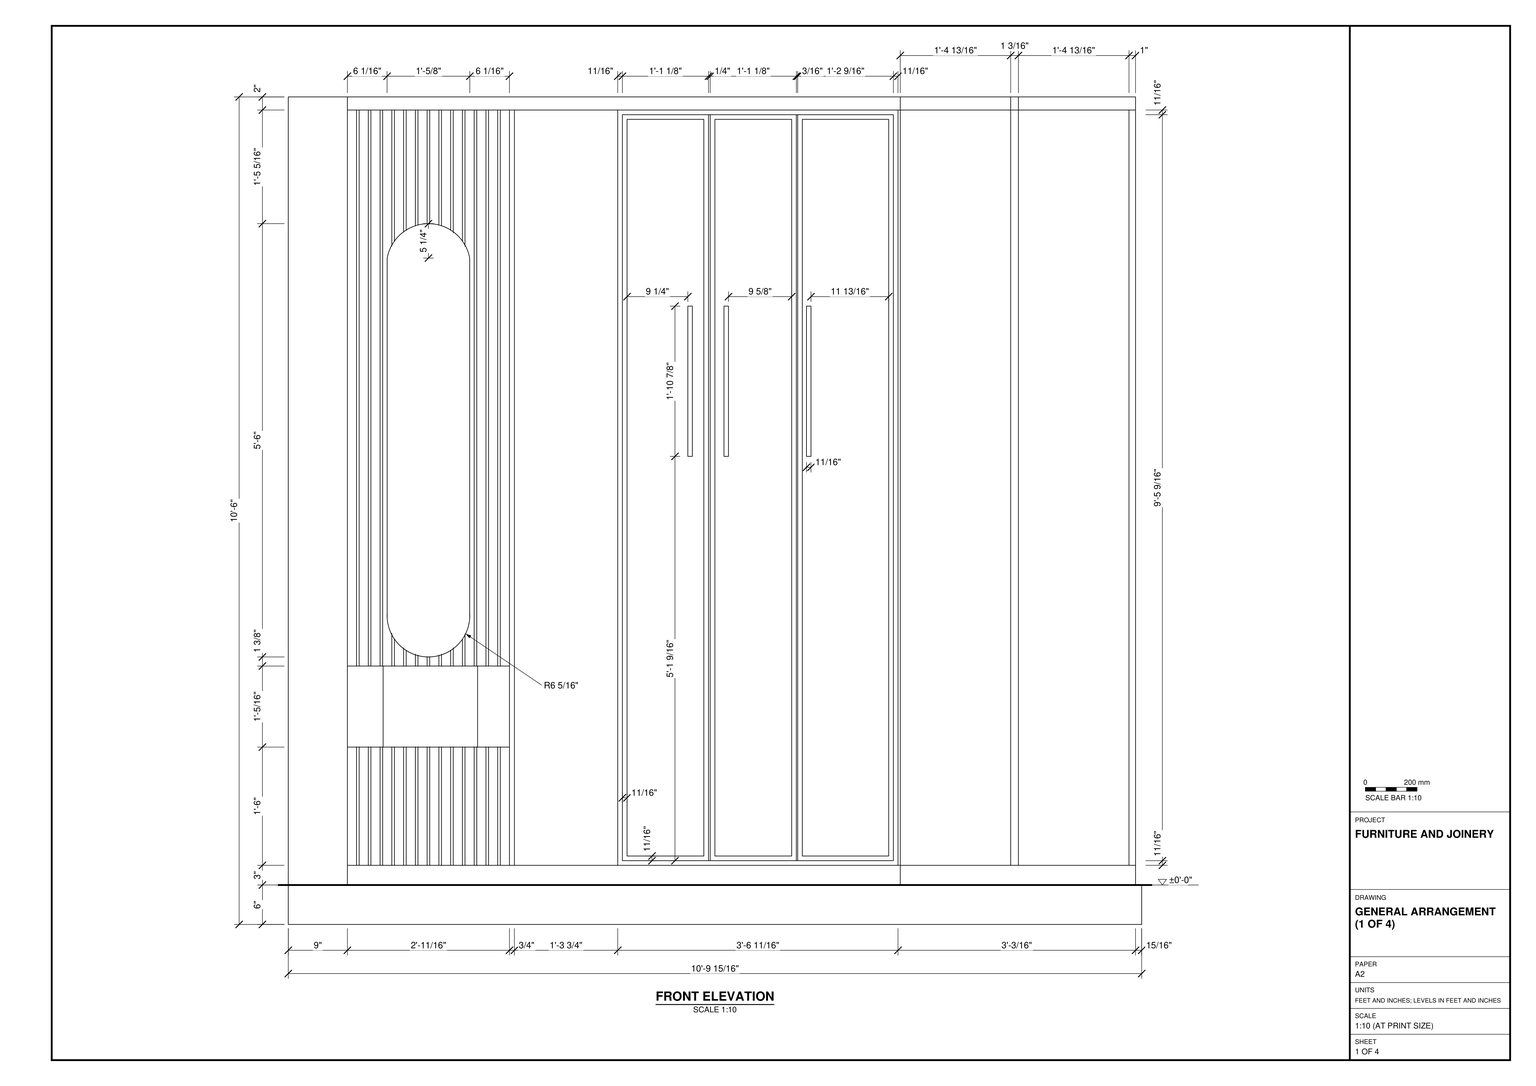
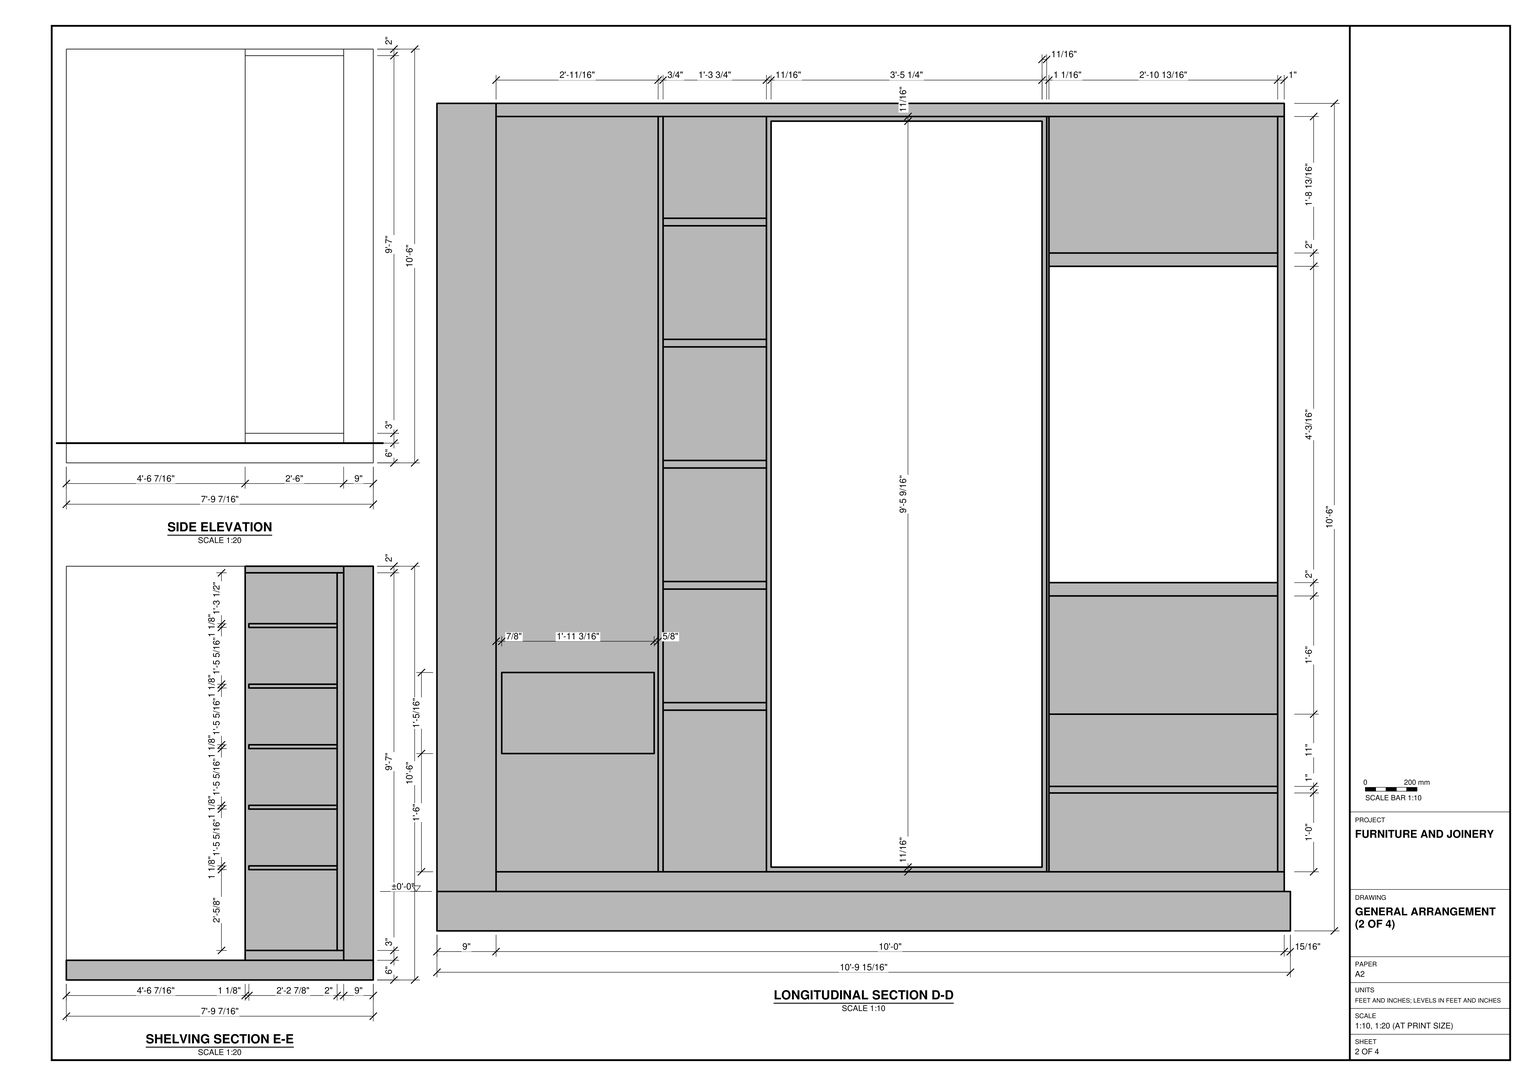
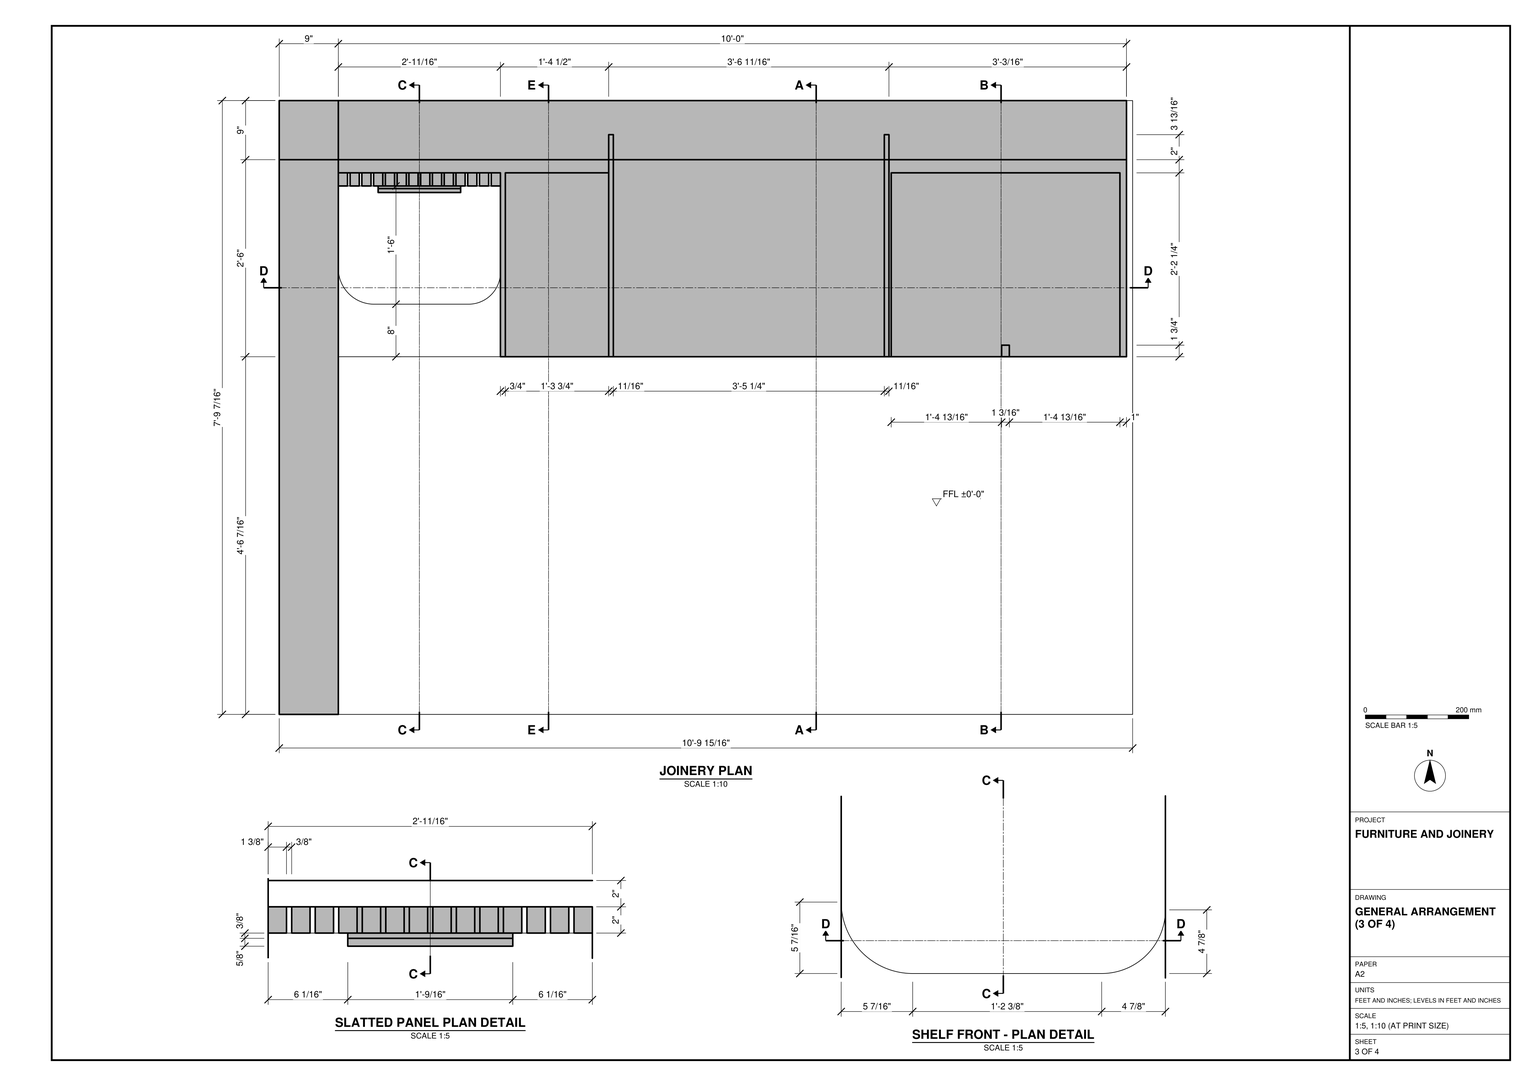
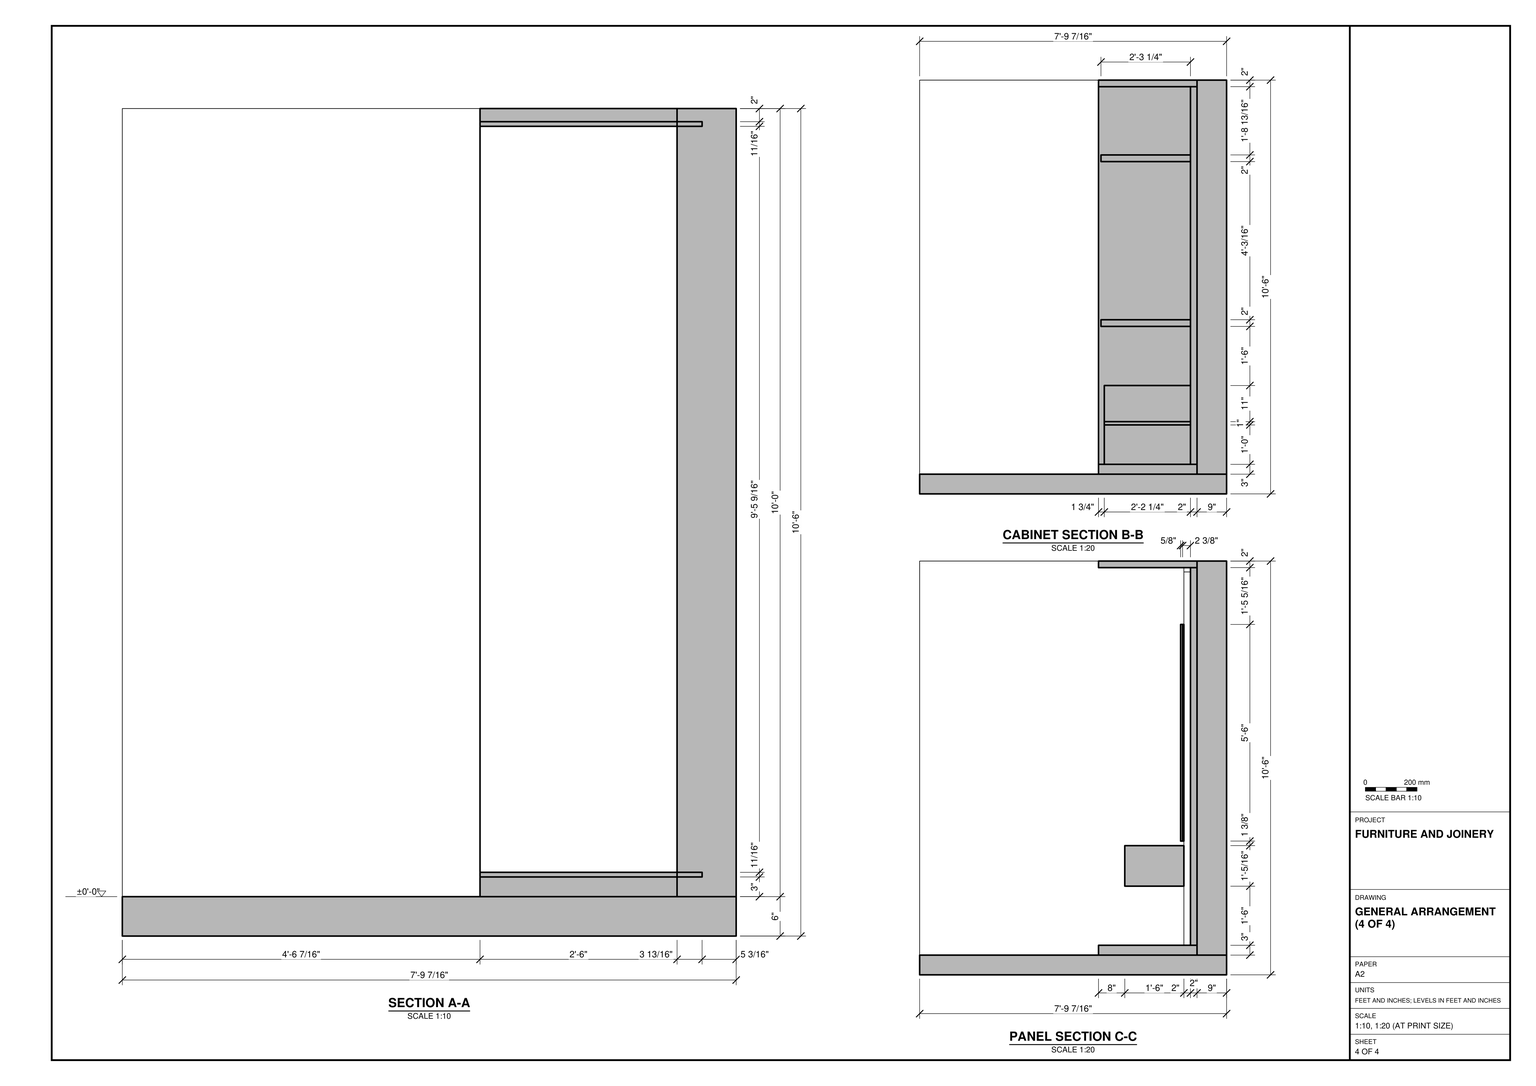
Build the wardrobe and its surrounding wall corner in SketchUp using task_files/diagram_01.pdf. Work in feet and inches, with the finished floor at ±0'-0". Including the floor slab and walls, the model measures 10'-9 15/16" wide, 7'-9 7/16" deep and 10'-6" high. Model the 6" floor slab and the 9" rear and left walls. Set the 10'-0" joinery run against the rear wall, starting at the inside face of the left wall, and leave the floor in front clear as shown in plan.

Build the continuous plinth and top panel. At the left end, centre the tall, round-ended mirror on the vertical slats. Fit the projecting shelf below it, following the plan detail for its rounded front corners. Between the mirror bay and the three framed wardrobe doors, build the narrow stack of shelves shown in section. Match the position of each door pull to the front elevation. In the right-hand bay, follow the elevation for the front divisions and the longitudinal section for the internal compartments.

Keep the slab, walls and distinct joinery pieces in separate groups or components, and use components for repeated parts. Any decor or loose items shown may be represented by suitable library components. Save one SketchUp model as output_files/wardrobe_with_shelving_and_mirrored_dressing_bay.skp.

# SketchUp Ruby script. Lengths in inches.
U = 1.inch
M = Sketchup.active_model
def pt(a) = Geom::Point3d.new(a.map { |v| v * U })
def face(e, loops, mat)
  f = e.add_face(loops[0].map { |a| pt(a) })
  loops[1..].each { |l| e.add_face(l.map { |a| pt(a) }).erase! }
  f.material = f.back_material = mat if mat
  f
end
# faces: each face lists its corners as indices into pts; further lists are holes
def faces(e, pts, list, mat = nil) = list.each { |f| face(e, (f[0].is_a?(Array) ? f : [f]).map { |l| l.map { |i| pts[i] } }, mat) }
# xy, xz, yz: faces in a plane at the given z, y or x. An outline is a flat list of corners, or four numbers for a rectangle; further outlines are holes
def ring(l) = l.size == 4 ? [[l[0], l[1]], [l[2], l[1]], [l[2], l[3]], [l[0], l[3]]] : l.each_slice(2).to_a
def flat(e, list, mat, &to3) = list.each { |f| face(e, (f[0].is_a?(Array) ? f : [f]).map { |l| ring(l).map { |u, v| to3.(u, v) } }, mat) }
def xy(e, z, list, mat = nil) = flat(e, list, mat) { |x, y| [x, y, z] }
def xz(e, y, list, mat = nil) = flat(e, list, mat) { |x, z| [x, y, z] }
def yz(e, x, list, mat = nil) = flat(e, list, mat) { |y, z| [x, y, z] }
def lines(e, pts, list) = list.each { |a, b| e.add_line(pt(pts[a]), pt(pts[b])) }
# prism: a flat outline (further loops are holes) pulled along v
def prism(e, loops, v, mat = nil)
  f = face(e, loops, mat); d = Geom::Vector3d.new(v.map { |x| x * U })
  f.pushpull(f.normal.samedirection?(d) ? d.length : -d.length)
end
def box(e, o, s, mat = nil) = prism(e, [[o, [o[0] + s[0], o[1], o[2]], [o[0] + s[0], o[1] + s[1], o[2]], [o[0], o[1] + s[1], o[2]]]], [0, 0, s[2]], mat)
def at(x, y, z, deg = 0) = Geom::Transformation.translation(pt([x, y, z])) * Geom::Transformation.rotation(ORIGIN, Z_AXIS, deg.degrees)
def axes(o, x, y, z) = Geom::Transformation.new([*x, 0, *y, 0, *z, 0, *pt(o).to_a, 1])
def part(name) = M.definitions.add(name)
# library, detail: a bought-in or finely detailed component or shape, given as its bounding box
def library(name, o, s) = part(name).tap { |d| box(d.entities, o, s) }
def detail(e, o, s) = box(e.add_group.entities, o, s)
def put(e, d, t, mat = nil) = e.add_instance(d, t).tap { |i| i.material = mat if mat }
def group(e, t, mat = nil) = e.add_group.tap { |g| g.transformation = t; g.material = mat if mat }.entities
root = M.entities
M.materials.add("[Color E01]").color = [255, 255, 204]
M.materials.add("[Color E03]").color = [255, 255, 101]
M.materials.add("[Color G01]").color = [204, 255, 204]
M.materials.add("[Metal Steel Textured]").color = [106, 110, 123]
M.materials.add("[Translucent Glass Gray]").color = [128, 128, 128]
M.materials["[Translucent Glass Gray]"].alpha = 0.5
c1 = part("Wardrobe shelf")
box(c1.entities,[0,-26.875,0],[15.73,26.875,1.15],"[Color E01]")
c2 = part("Wardrobe upright")
prism(c2.entities,[[[0,0,115],[1.4,0,115],[1.4,0,113.6875],[1.4,0,0],[0,0,0]]],[0,-2,0],"[Color E01]")
c3 = part("Group\#10")
xz(c3.entities,0,[[0,0,0.6875,22.875]])
c4 = library("Group\#11",[-0.02,-1,-1.38],[12.6,1,65.97])
g1 = group(root,at(3.61,0,0))
box(g1,[-3.61,0,0],[129.94,93.46,6])
g2 = group(root,at(9,84.46,6))
xy(g2,0,[[-9,-84.46,0,0],[-9,0,0,9],[0,0,120,9]])
xy(g2,120,[[-9,-84.46,0,0],[-9,0,0,9],[0,0,120,9]])
xz(g2,-84.46,[[-9,0,0,120]])
xz(g2,0,[[-9,0,0,120],[0,0,120,120]])
xz(g2,9,[[-9,0,0,120],[0,0,120,120]])
yz(g2,-9,[[-84.46,0,0,120],[0,0,9,120]])
yz(g2,0,[[-84.46,0,0,120],[0,0,9,120]])
yz(g2,120,[[0,0,9,120]])
g3 = group(root,at(9,60.46,6),"[Color E01]")
xy(g3,0,[[0,-6,120,24]],"[Color E03]")
xy(g3,3,[[100.99,-6,102.16,-4.24]])
xy(g3,3,[[0,-6,24.68,22],[25.43,-6,41.16,22],[41.16,24,83.84,27.8125]],"[Color E01]")
xy(g3,3,[[24.68,-6,25.43,-6,25.43,22,41.16,22,41.16,24,0,24,0,22,24.68,22],[41.16,-6,83.84,24],[83.84,-6,84.18,-6,84.18,22,119,22,119,-6,120,-6,120,24,83.84,24],[84.18,-6,100.99,-4.24],[102.16,-6,119,-4.24]],"[Color E03]")
xy(g3,3.71,[[41.87,-6,83.125,27.8125]],"[Color E01]")
xy(g3,117.29,[[41.87,-6,83.125,27.8125]],"[Color E01]")
xy(g3,118,[[0,-6,24.68,22],[25.43,-6,41.16,22],[84.18,-6,84.18,22,119,22,119,-6,102.16,-6,102.16,-4.24,100.99,-4.24,100.99,-6],[41.16,24,83.84,27.8125]],"[Color E01]")
xy(g3,118,[[24.68,-6,24.68,22,0,22,0,24,41.16,24,41.16,22,25.43,22,25.43,-6],[41.16,-6,83.84,24],[83.84,-6,83.84,24,120,24,120,-6,119,-6,119,22,84.18,22,84.18,-6]],"[Color E03]")
xy(g3,120,[[0,-6,120,24]],"[Color E01]")
xz(g3,-6,[[0,0,84.18,3],[84.18,0,120,3],[24.68,3,25.43,118],[[41.16,3,83.84,118],[54.98,3.71,83.125,117.29]],[83.84,3,84.18,118],
  [119,3,120,118],[54.98,3.71,83.125,117.29],[0,118,84.18,120],[84.18,118,100.99,120],[100.99,118,102.16,120],
  [102.16,118,120,120]],"[Color E01]")
xz(g3,-6,[[100.99,3,102.16,118]],"[Metal Steel Textured]")
xz(g3,-6,[[25.43,3,41.16,118],[84.18,3,100.99,118],[102.16,3,119,118]],"[Translucent Glass Gray]")
xz(g3,-4.24,[[100.99,3,102.16,118]],"[Color E03]")
xz(g3,22,[[0,3,23.28,118],[25.43,3,41.16,101.36],[84.18,3,119,45],[84.18,47.03,119,118],[25.43,102.51,41.16,118]],"[Color E01]")
xz(g3,24,[[0,0,120,3],[0,3,120,118],[0,118,120,120]],"[Color E03]")
xz(g3,27.8125,[[[41.16,3,83.84,118],[41.87,3.71,83.125,117.29]]],"[Color E01]")
yz(g3,0,[[-6,0,24,3],[22,3,24,118],[-6,118,24,120]],"[Color E01]")
yz(g3,24.68,[[-6,3,22,116.6875],[-6,116.6875,22,118]],"[Color E01]")
yz(g3,25.43,[[-6,3,22,118]],"[Color E01]")
yz(g3,41.16,[[-6,3,22,118],[22,3,27.8125,118]],"[Color E01]")
yz(g3,41.87,[[-6,3.71,27.8125,117.29]],"[Color E01]")
yz(g3,83.125,[[-6,3.71,27.8125,117.29]],"[Color E01]")
yz(g3,83.84,[[-6,3,27.8125,118]],"[Color E01]")
yz(g3,84.18,[[-6,3,22,118]],"[Color E01]")
yz(g3,100.99,[[-6,3,-4.24,118]],"[Color E03]")
yz(g3,102.16,[[-6,3,-4.24,118]],"[Color E03]")
yz(g3,119,[[-6,3,22,118]],"[Color E01]")
yz(g3,120,[[-6,3,24,118],[-6,118,24,120]],"[Color E01]")
yz(g3,120,[[-6,0,24,3]],"[Color E03]")
put(g3,c1,at(25.43,22,101.36))
put(g3,c1,at(25.43,22,82.92))
put(g3,c1,at(25.43,22,64.48))
put(g3,c1,at(25.43,22,46.04))
put(g3,c1,at(25.43,22,27.61))
put(g3,c2,at(23.28,22,3))
put(g3,c2,at(21.49,22,3))
put(g3,c2,at(19.7,22,3))
put(g3,c2,at(17.91,22,3))
put(g3,c2,at(16.12,22,3))
put(g3,c2,at(14.33,22,3))
put(g3,c2,at(12.54,22,3))
put(g3,c2,at(10.75,22,3))
put(g3,c2,at(8.95,22,3))
put(g3,c2,at(7.16,22,3))
put(g3,c2,at(5.37,22,3))
put(g3,c2,at(3.58,22,3))
put(g3,c2,at(1.79,22,3))
put(g3,c2,at(0,22,3))
g4 = group(g3,at(84.18,-4.24,3),"[Color E01]")
xy(g4,0,[[0,0,34.82,26.24]])
xy(g4,12,[[0,0,34.82,26.24]])
xy(g4,13,[[0,0,34.82,26.24]])
xy(g4,24,[[0,0,34.82,26.24]])
xz(g4,0,[[0,0,34.82,12],[0,12,34.82,13],[0,13,34.82,24]])
xz(g4,26.24,[[0,0,34.82,12],[0,12,34.82,13],[0,13,34.82,24]])
yz(g4,0,[[0,0,26.24,12],[0,12,26.24,13],[0,13,26.24,24]])
yz(g4,34.82,[[0,0,26.24,12],[0,12,26.24,13],[0,13,26.24,24]])
g5 = group(g3,at(84.18,22,45),"[Color E01]")
xy(g5,0,[[0,-27.25,34.82,0]],"[Color G01]")
xy(g5,2.03,[[0,-27.25,34.82,0]],"[Color E01]")
xz(g5,-27.25,[[0,0,34.82,2.03]],"[Color E01]")
xz(g5,0,[[0,0,34.82,2.03]],"[Color G01]")
yz(g5,0,[[-27.25,0,0,2.03]],"[Color G01]")
yz(g5,34.82,[[-27.25,0,0,2.03]],"[Color G01]")
g6 = group(g3,at(84.18,22,95.1875),"[Color E01]")
box(g6,[0,-27.25,0],[34.82,27.25,2.03],"[Color E01]")
put(g3,c3,at(51.83,-6,65.27))
put(g3,c3,at(57.33,-6,65.27))
put(g3,c3,at(69.9,-6,65.27))
g7 = group(g3,at(41.87,-6,3.71))
xz(g7,0,[[[0,0,13.11,113.58],[0.71,0.71,12.4,112.875]],[0.71,0.71,12.4,112.875]],"[Color E01]")
g8 = group(g3,at(55.25,-6,3.71))
xz(g8,0,[[[0,0,13.11,113.58],[0.71,0.71,12.4,112.875]],[0.71,0.71,12.4,112.875]],"[Color E01]")
g9 = group(g3,at(68.56,-6,3.71))
xz(g9,0,[[[0,0,14.57,113.58],[0.71,0.71,13.86,112.875]],[0.71,0.71,13.86,112.875]],"[Color E01]")
put(g3,c4,at(6.06,20,36.11))
g10 = group(g3,at(0,20,21))
prism(g10,[[[0,0,0],[24.68,0,0],[24.68,-13.15,0],[24.68,-13.3,0],[24.67,-13.45,0],[24.66,-13.6,0],[24.64,-13.76,0],[24.62,-13.91,0],[24.59,-14.06,0],[24.5625,-14.21,0],[24.53,-14.35,0],[24.49,-14.5,0],[24.44,-14.65,0],[24.39,-14.79,0],[24.34,-14.93,0],[24.28,-15.07,0],[24.22,-15.21,0],[24.15,-15.35,0],[24.08,-15.49,0],[24,-15.62,0],[23.92,-15.75,0],[23.84,-15.875,0],[23.75,-16,0],[23.66,-16.12,0],[23.57,-16.24,0],[23.47,-16.36,0],[23.36,-16.47,0],[23.26,-16.58,0],[23.15,-16.68,0],[23.04,-16.79,0],[22.92,-16.89,0],[22.8,-16.98,0],[22.68,-17.07,0],[22.55,-17.16,0],[22.43,-17.24,0],[22.3,-17.32,0],[22.16,-17.4,0],[22.03,-17.47,0],[21.89,-17.54,0],[21.75,-17.6,0],[21.61,-17.66,0],[21.47,-17.71,0],[21.33,-17.76,0],[21.18,-17.81,0],[21.03,-17.85,0],[20.88,-17.88,0],[20.74,-17.91,0],[20.59,-17.94,0],[20.43,-17.96,0],[20.28,-17.98,0],[20.13,-17.99,0],[19.98,-18,0],[19.83,-18,0],[5.44,-18,0],[5.27,-18,0],[5.1,-17.99,0],[4.93,-17.98,0],[4.76,-17.96,0],[4.59,-17.93,0],[4.42,-17.9,0],[4.25,-17.87,0],[4.09,-17.83,0],[3.92,-17.78,0],[3.76,-17.73,0],[3.6,-17.68,0],[3.4375,-17.62,0],[3.28,-17.55,0],[3.125,-17.48,0],[2.97,-17.41,0],[2.82,-17.33,0],[2.67,-17.24,0],[2.53,-17.15,0],[2.38,-17.06,0],[2.24,-16.96,0],[2.11,-16.86,0],[1.97,-16.75,0],[1.84,-16.64,0],[1.72,-16.53,0],[1.59,-16.41,0],[1.47,-16.28,0],[1.36,-16.16,0],[1.25,-16.03,0],[1.14,-15.89,0],[1.04,-15.76,0],[0.94,-15.62,0],[0.85,-15.47,0],[0.76,-15.33,0],[0.67,-15.18,0],[0.59,-15.03,0],[0.52,-14.875,0],[0.45,-14.72,0],[0.38,-14.5625,0],[0.32,-14.4,0],[0.27,-14.24,0],[0.22,-14.08,0],[0.17,-13.91,0],[0.13,-13.75,0],[0.1,-13.58,0],[0.07,-13.41,0],[0.04,-13.24,0],[0.02,-13.07,0],[0.01,-12.9,0],[0,-12.73,0],[0,-12.56,0]]],[0,0,12.34])
